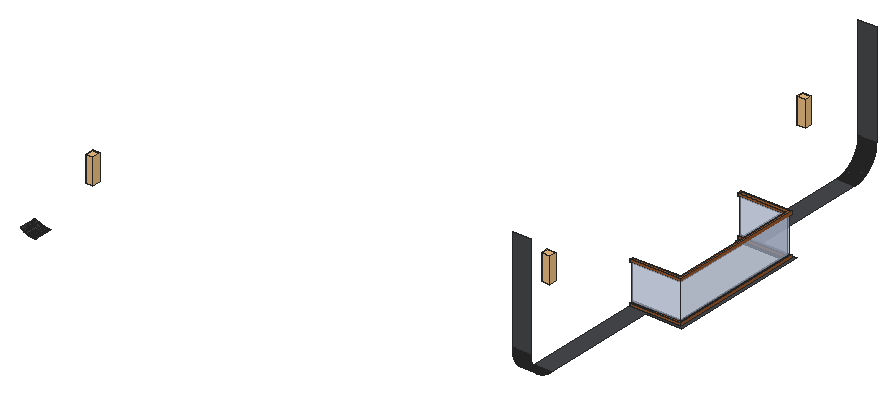
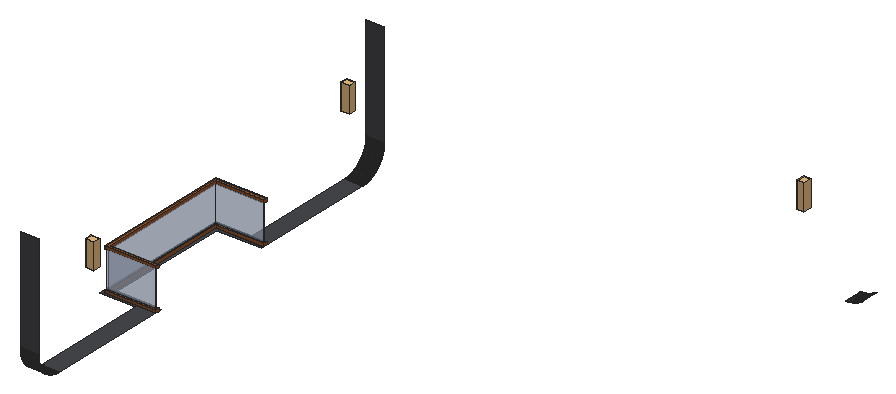
# SketchUp Ruby script. Lengths in inches.
U = 1.inch
M = Sketchup.active_model
def pt(a) = Geom::Point3d.new(a.map { |v| v * U })
def face(e, loops, mat)
  f = e.add_face(loops[0].map { |a| pt(a) })
  loops[1..].each { |l| e.add_face(l.map { |a| pt(a) }).erase! }
  f.material = f.back_material = mat if mat
  f
end
# faces: each face lists its corners as indices into pts; further lists are holes
def faces(e, pts, list, mat = nil) = list.each { |f| face(e, (f[0].is_a?(Array) ? f : [f]).map { |l| l.map { |i| pts[i] } }, mat) }
# xy, xz, yz: faces in a plane at the given z, y or x. An outline is a flat list of corners, or four numbers for a rectangle; further outlines are holes
def ring(l) = l.size == 4 ? [[l[0], l[1]], [l[2], l[1]], [l[2], l[3]], [l[0], l[3]]] : l.each_slice(2).to_a
def flat(e, list, mat, &to3) = list.each { |f| face(e, (f[0].is_a?(Array) ? f : [f]).map { |l| ring(l).map { |u, v| to3.(u, v) } }, mat) }
def xy(e, z, list, mat = nil) = flat(e, list, mat) { |x, y| [x, y, z] }
def xz(e, y, list, mat = nil) = flat(e, list, mat) { |x, z| [x, y, z] }
def yz(e, x, list, mat = nil) = flat(e, list, mat) { |y, z| [x, y, z] }
def lines(e, pts, list) = list.each { |a, b| e.add_line(pt(pts[a]), pt(pts[b])) }
# prism: a flat outline (further loops are holes) pulled along v
def prism(e, loops, v, mat = nil)
  f = face(e, loops, mat); d = Geom::Vector3d.new(v.map { |x| x * U })
  f.pushpull(f.normal.samedirection?(d) ? d.length : -d.length)
end
def box(e, o, s, mat = nil) = prism(e, [[o, [o[0] + s[0], o[1], o[2]], [o[0] + s[0], o[1] + s[1], o[2]], [o[0], o[1] + s[1], o[2]]]], [0, 0, s[2]], mat)
def at(x, y, z, deg = 0) = Geom::Transformation.translation(pt([x, y, z])) * Geom::Transformation.rotation(ORIGIN, Z_AXIS, deg.degrees)
def axes(o, x, y, z) = Geom::Transformation.new([*x, 0, *y, 0, *z, 0, *pt(o).to_a, 1])
def part(name) = M.definitions.add(name)
# library, detail: a bought-in or finely detailed component or shape, given as its bounding box
def library(name, o, s) = part(name).tap { |d| box(d.entities, o, s) }
def detail(e, o, s) = box(e.add_group.entities, o, s)
def put(e, d, t, mat = nil) = e.add_instance(d, t).tap { |i| i.material = mat if mat }
def group(e, t, mat = nil) = e.add_group.tap { |g| g.transformation = t; g.material = mat if mat }.entities
root = M.entities
M.materials.add("1432 AP 8245 TAR ROAD").color = [71, 72, 75]
M.materials.add("[Translucent Glass Blue]").color = [195, 208, 233]
M.materials["[Translucent Glass Blue]"].alpha = 0.5
M.materials.add("[Wood Cherry Original]").color = [152, 86, 42]
c1 = library("WALL LIGHT 69",[4.19,4.05,-8.78],[4.61,5.7,17.13])
c2 = part("Group\#47")
xy(c2.entities,0,[[0,0,0,2,32,2,32,90,0,90,0,92,34,92,34,0]])
xy(c2.entities,1.75,[[0.75,0.75,33.25,0.75,33.25,91.25,0.75,91.25,0.75,90.75,32.75,90.75,32.75,1.25,0.75,1.25]])
xy(c2.entities,2,[[[0,0,34,0,34,92,0,92,0,90,32,90,32,2,0,2],[0.75,0.75,0.75,1.25,32.75,1.25,32.75,90.75,0.75,90.75,0.75,91.25,33.25,91.25,33.25,0.75]]])
xy(c2.entities,26,[[[0,0,0,2,32,2,32,90,0,90,0,92,34,92,34,0],[0.75,0.75,33.25,0.75,33.25,91.25,0.75,91.25,0.75,90.75,32.75,90.75,32.75,1.25,0.75,1.25]]])
xy(c2.entities,26.25,[[0.75,0.75,0.75,1.25,32.75,1.25,32.75,90.75,0.75,90.75,0.75,91.25,33.25,91.25,33.25,0.75]])
xy(c2.entities,28,[[0,0,34,0,34,92,0,92,0,90,32,90,32,2,0,2]])
xz(c2.entities,0,[[0,0,34,2],[0,26,34,28]])
xz(c2.entities,0.75,[[0.75,1.75,33.25,2],[0.75,26,33.25,26.25]])
xz(c2.entities,1.25,[[0.75,1.75,32.75,2],[0.75,26,32.75,26.25]])
xz(c2.entities,2,[[0,0,32,2],[0,26,32,28]])
xz(c2.entities,90,[[0,0,32,2],[0,26,32,28]])
xz(c2.entities,90.75,[[0.75,1.75,32.75,2],[0.75,26,32.75,26.25]])
xz(c2.entities,91.25,[[0.75,1.75,33.25,2],[0.75,26,33.25,26.25]])
xz(c2.entities,92,[[0,0,34,2],[0,26,34,28]])
yz(c2.entities,0,[[0,0,2,2],[90,0,92,2],[0,26,2,28],[90,26,92,28]])
yz(c2.entities,0.75,[[0.75,1.75,1.25,2],[90.75,1.75,91.25,2],[0.75,26,1.25,26.25],[90.75,26,91.25,26.25]])
yz(c2.entities,32,[[2,0,90,2],[2,26,90,28]])
yz(c2.entities,32.75,[[1.25,1.75,90.75,2],[1.25,26,90.75,26.25]])
yz(c2.entities,33.25,[[0.75,1.75,91.25,2],[0.75,26,91.25,26.25]])
yz(c2.entities,34,[[0,0,92,2],[0,26,92,28]])
g1 = group(c2.entities,at(0.75,0.75,1.75),"[Translucent Glass Blue]")
prism(g1,[[[32,90,0],[0,90,0],[0,90.5,0],[32.5,90.5,0],[32.5,0,0],[0,0,0],[0,0.5,0],[32,0.5,0]]],[0,0,24.5])
xy(root,455.79,[[573,161.13,585,161.37],[573,161.37,585,161.37,585,239.37,609,239.37,609,335.37,585,335.37,585,413.37,573,413.37,573,329.37,603,329.37,603,245.37,573,245.37],[573,413.37,585,413.61]],"1432 AP 8245 TAR ROAD")
xy(root,461.79,[[293.76,95.37,294,107.37]],"1432 AP 8245 TAR ROAD")
xz(root,143.37,[[573,473.56,585,473.79],[573,473.79,585,542.79]],"1432 AP 8245 TAR ROAD")
xz(root,431.36,[[573,473.09,585,473.32]],"1432 AP 8245 TAR ROAD")
xz(root,431.37,[[573,473.56,585,473.79],[573,473.79,585,542.79]],"1432 AP 8245 TAR ROAD")
p = [[573,159.96,455.85],[573,159.72,455.87],[585,159.72,455.87],[585,159.96,455.85],[573,160.19,455.83],[585,160.19,455.83],
  [573,160.43,455.82],[585,160.43,455.82],[573,160.66,455.81],[585,160.66,455.81],[573,160.9,455.8],[585,160.9,455.8],
  [573,161.13,455.79],[585,161.13,455.79],[573,413.84,455.8],[573,413.61,455.79],[585,413.61,455.79],[585,413.84,455.8],
  [573,414.08,455.81],[585,414.08,455.81],[573,414.3125,455.82],[585,414.3125,455.82],[573,414.55,455.83],[585,414.55,455.83],
  [573,414.78,455.85],[585,414.78,455.85],[573,415.02,455.87],[585,415.02,455.87],[573,159.02,455.95],[573,158.79,455.98],
  [585,158.79,455.98],[585,159.02,455.95],[573,159.25,455.92],[585,159.25,455.92],[573,159.49,455.89],[585,159.49,455.89],
  [573,415.25,455.89],[585,415.25,455.89],[573,415.49,455.92],[585,415.49,455.92],[573,415.72,455.95],[585,415.72,455.95],
  [573,415.95,455.98],[585,415.95,455.98],[573,158.55,456.01],[573,158.32,456.05],[585,158.32,456.05],[585,158.55,456.01],
  [573,416.1875,456.01],[585,416.1875,456.01],[573,416.42,456.05],[585,416.42,456.05],[573,157.86,456.14],[573,157.63,456.19],
  [585,157.63,456.19],[585,157.86,456.14],[573,158.09,456.09],[585,158.09,456.09],[573,416.65,456.09],[585,416.65,456.09],
  [573,416.88,456.14],[585,416.88,456.14],[573,417.11,456.19],[585,417.11,456.19],[573,157.4,456.24],[573,157.17,456.29],
  [585,157.17,456.29],[585,157.4,456.24],[573,417.34,456.24],[585,417.34,456.24],[573,417.57,456.29],[585,417.57,456.29],
  [573,156.9375,456.35],[573,156.71,456.41],[585,156.71,456.41],[585,156.9375,456.35],[573,417.8,456.35],[585,417.8,456.35],
  [573,418.03,456.41],[585,418.03,456.41],[573,156.48,456.47],[585,156.48,456.47],[573,418.26,456.47],[585,418.26,456.47],
  [573,156.26,456.53],[573,156.03,456.6],[585,156.03,456.6],[585,156.26,456.53],[573,418.48,456.53],[585,418.48,456.53],
  [573,418.71,456.6],[585,418.71,456.6],[573,155.81,456.67],[585,155.81,456.67],[573,418.93,456.67],[585,418.93,456.67],
  [573,155.58,456.75],[573,155.36,456.82],[585,155.36,456.82],[585,155.58,456.75],[573,419.16,456.75],[585,419.16,456.75],
  [573,419.38,456.82],[585,419.38,456.82],[573,155.14,456.9],[585,155.14,456.9],[573,419.6,456.9],[585,419.6,456.9],
  [573,154.92,456.99],[585,154.92,456.99],[573,419.82,456.99],[585,419.82,456.99],[573,154.7,457.07],[585,154.7,457.07],
  [573,420.04,457.07],[585,420.04,457.07],[573,154.48,457.16],[585,154.48,457.16],[573,420.26,457.16],[585,420.26,457.16],
  [573,154.26,457.25],[585,154.26,457.25],[573,420.48,457.25],[585,420.48,457.25],[573,154.05,457.35],[573,153.83,457.45],
  [585,153.83,457.45],[585,154.05,457.35],[573,420.69,457.35],[585,420.69,457.35],[573,420.91,457.45],[585,420.91,457.45],
  [573,153.62,457.55],[585,153.62,457.55],[573,421.12,457.55],[585,421.12,457.55],[573,153.41,457.65],[585,153.41,457.65],
  [573,421.33,457.65],[585,421.33,457.65],[573,153.2,457.75],[585,153.2,457.75],[573,421.54,457.75],[585,421.54,457.75],
  [573,152.99,457.86],[585,152.99,457.86],[573,421.75,457.86],[585,421.75,457.86],[573,152.78,457.97],[585,152.78,457.97],
  [573,421.96,457.97],[585,421.96,457.97],[573,152.57,458.09],[585,152.57,458.09],[573,422.17,458.09],[585,422.17,458.09],
  [573,152.37,458.2],[585,152.37,458.2],[573,422.37,458.2],[585,422.37,458.2],[573,152.17,458.32],[585,152.17,458.32],
  [573,422.57,458.32],[585,422.57,458.32],[573,151.96,458.44],[585,151.96,458.44],[573,422.77,458.44],[585,422.77,458.44],
  [573,151.76,458.57],[585,151.76,458.57],[573,422.97,458.57],[585,422.97,458.57],[573,151.57,458.7],[585,151.57,458.7],
  [573,423.17,458.7],[585,423.17,458.7],[573,151.37,458.83],[585,151.37,458.83],[573,423.37,458.83],[585,423.37,458.83],
  [573,151.17,458.96],[585,151.17,458.96],[573,423.57,458.96],[585,423.57,458.96],[573,150.98,459.09],[585,150.98,459.09],
  [573,423.76,459.09],[585,423.76,459.09],[573,150.79,459.23],[585,150.79,459.23],[573,423.95,459.23],[585,423.95,459.23],
  [573,150.6,459.37],[585,150.6,459.37],[573,424.14,459.37],[585,424.14,459.37],[573,150.41,459.51],[585,150.41,459.51],
  [573,424.33,459.51],[585,424.33,459.51],[573,150.23,459.66],[585,150.23,459.66],[573,424.51,459.66],[585,424.51,459.66],
  [573,150.04,459.8],[585,150.04,459.8],[573,424.7,459.8],[585,424.7,459.8],[573,149.86,459.95],[585,149.86,459.95],
  [573,424.88,459.95],[585,424.88,459.95],[573,149.68,460.1],[585,149.68,460.1],[573,425.06,460.1],[585,425.06,460.1],
  [573,149.5,460.26],[585,149.5,460.26],[573,425.24,460.26],[585,425.24,460.26],[573,149.33,460.42],[585,149.33,460.42],
  [573,425.41,460.42],[585,425.41,460.42],[573,149.15,460.57],[585,149.15,460.57],[573,425.59,460.57],[585,425.59,460.57],
  [573,148.98,460.74],[585,148.98,460.74],[573,425.76,460.74],[585,425.76,460.74],[573,148.81,460.9],[585,148.81,460.9],
  [573,425.93,460.9],[585,425.93,460.9],[573,148.64,461.0625],[585,148.64,461.0625],[573,426.1,461.0625],[585,426.1,461.0625],
  [573,148.48,461.23],[585,148.48,461.23],[573,426.26,461.23],[585,426.26,461.23],[573,148.3125,461.4],[585,148.3125,461.4],
  [573,426.43,461.4],[585,426.43,461.4],[573,148.15,461.57],[585,148.15,461.57],[573,426.59,461.57],[585,426.59,461.57],
  [573,147.99,461.75],[585,147.99,461.75],[573,426.75,461.75],[585,426.75,461.75],[573,147.84,461.92],[585,147.84,461.92],
  [573,426.9,461.92],[585,426.9,461.92],[292.59,107.37,461.85],[292.35,107.37,461.87],[292.35,95.37,461.87],[292.59,95.37,461.85],
  [292.82,107.37,461.83],[292.82,95.37,461.83],[293.06,107.37,461.82],[293.06,95.37,461.82],[293.29,107.37,461.81],[293.29,95.37,461.81],
  [293.53,107.37,461.8],[293.53,95.37,461.8],[293.76,107.37,461.79],[293.76,95.37,461.79],[291.65,107.37,461.95],[291.42,107.37,461.98],
  [291.42,95.37,461.98],[291.65,95.37,461.95],[291.88,107.37,461.92],[291.88,95.37,461.92],[292.12,107.37,461.89],[292.12,95.37,461.89],
  [573,147.68,462.1],[585,147.68,462.1],[573,427.06,462.1],[585,427.06,462.1],[291.18,107.37,462.01],[290.95,107.37,462.05],
  [290.95,95.37,462.05],[291.18,95.37,462.01],[290.49,107.37,462.14],[290.26,107.37,462.19],[290.26,95.37,462.19],[290.49,95.37,462.14],
  [290.72,107.37,462.09],[290.72,95.37,462.09],[573,147.53,462.28],[585,147.53,462.28],[573,427.21,462.28],[585,427.21,462.28],
  [290.03,107.37,462.24],[289.8,107.37,462.29],[289.8,95.37,462.29],[290.03,95.37,462.24],[289.57,107.37,462.35],[289.34,107.37,462.41],
  [289.34,95.37,462.41],[289.57,95.37,462.35],[573,147.38,462.46],[585,147.38,462.46],[573,427.36,462.46],[585,427.36,462.46],
  [289.11,107.37,462.47],[289.11,95.37,462.47],[288.89,107.37,462.53],[288.66,107.37,462.6],[288.66,95.37,462.6],[288.89,95.37,462.53],
  [573,147.23,462.65],[585,147.23,462.65],[573,427.51,462.65],[585,427.51,462.65],[288.4375,107.37,462.67],[288.4375,95.37,462.67],
  [573,147.09,462.83],[585,147.09,462.83],[573,427.65,462.83],[585,427.65,462.83],[288.21,107.37,462.75],[287.99,107.37,462.82],
  [287.99,95.37,462.82],[288.21,95.37,462.75],[287.77,107.37,462.9],[287.77,95.37,462.9],[573,146.95,463.02],[585,146.95,463.02],
  [573,427.79,463.02],[585,427.79,463.02],[287.55,107.37,462.99],[287.55,95.37,462.99],[287.33,107.37,463.07],[287.33,95.37,463.07],
  [573,146.81,463.21],[585,146.81,463.21],[573,427.93,463.21],[585,427.93,463.21],[287.11,107.37,463.16],[287.11,95.37,463.16],
  [286.89,107.37,463.25],[286.89,95.37,463.25],[573,146.67,463.4],[585,146.67,463.4],[573,428.07,463.4],[585,428.07,463.4],
  [286.68,107.37,463.35],[286.46,107.37,463.45],[286.46,95.37,463.45],[286.68,95.37,463.35],[286.25,107.37,463.55],[286.25,95.37,463.55],
  [573,146.54,463.6],[585,146.54,463.6],[573,428.2,463.6],[585,428.2,463.6],[286.04,107.37,463.65],[286.04,95.37,463.65],
  [285.83,107.37,463.75],[285.83,95.37,463.75],[573,146.4,463.79],[585,146.4,463.79],[573,428.34,463.79],[585,428.34,463.79],
  [285.62,107.37,463.86],[285.62,95.37,463.86],[573,146.27,463.99],[585,146.27,463.99],[573,428.47,463.99],[585,428.47,463.99],
  [285.41,107.37,463.97],[285.41,95.37,463.97],[285.2,107.37,464.09],[285.2,95.37,464.09],[573,146.15,464.1875],[585,146.15,464.1875],
  [573,428.59,464.1875],[585,428.59,464.1875],[285,107.37,464.2],[285,95.37,464.2],[284.8,107.37,464.32],[284.8,95.37,464.32],
  [573,146.02,464.39],[585,146.02,464.39],[573,428.72,464.39],[585,428.72,464.39],[284.6,107.37,464.44],[284.6,95.37,464.44],
  [284.39,107.37,464.57],[284.39,95.37,464.57],[573,145.9,464.59],[585,145.9,464.59],[573,428.84,464.59],[585,428.84,464.59],
  [284.2,107.37,464.7],[284.2,95.37,464.7],[573,145.78,464.79],[585,145.78,464.79],[573,428.96,464.79],[585,428.96,464.79],
  [284,107.37,464.83],[284,95.37,464.83],[283.8,107.37,464.96],[283.8,95.37,464.96],[573,145.67,465],[585,145.67,465],
  [573,429.07,465],[585,429.07,465],[283.61,107.37,465.09],[283.61,95.37,465.09],[573,145.55,465.2],[585,145.55,465.2],
  [573,429.1875,465.2],[585,429.1875,465.2],[573,145.44,465.41],[585,145.44,465.41],[573,429.3,465.41],[585,429.3,465.41],
  [573,145.33,465.62],[585,145.33,465.62],[573,429.41,465.62],[585,429.41,465.62],[573,145.23,465.83],[585,145.23,465.83],
  [573,429.51,465.83],[585,429.51,465.83],[573,145.125,466.04],[585,145.125,466.04],[573,429.62,466.04],[585,429.62,466.04],
  [573,145.02,466.26],[585,145.02,466.26],[573,429.72,466.26],[585,429.72,466.26],[573,144.93,466.47],[585,144.93,466.47],
  [573,429.8125,466.47],[585,429.8125,466.47],[573,144.83,466.6875],[585,144.83,466.6875],[573,429.91,466.6875],[585,429.91,466.6875],
  [573,144.74,466.9],[585,144.74,466.9],[573,430,466.9],[585,430,466.9],[573,144.65,467.12],[585,144.65,467.12],
  [573,430.09,467.12],[585,430.09,467.12],[573,144.57,467.34],[585,144.57,467.34],[573,430.17,467.34],[585,430.17,467.34],
  [573,144.48,467.5625],[585,144.48,467.5625],[573,430.26,467.5625],[585,430.26,467.5625],[573,144.4,467.78],[585,144.4,467.78],
  [573,430.34,467.78],[585,430.34,467.78],[573,144.33,468.01],[585,144.33,468.01],[573,430.41,468.01],[585,430.41,468.01],
  [573,144.25,468.23],[585,144.25,468.23],[573,430.49,468.23],[585,430.49,468.23],[573,144.18,468.45],[585,144.18,468.45],
  [573,430.56,468.45],[585,430.56,468.45],[573,144.11,468.68],[585,144.11,468.68],[573,430.63,468.68],[585,430.63,468.68],
  [573,144.05,468.91],[585,144.05,468.91],[573,430.69,468.91],[585,430.69,468.91],[573,143.98,469.13],[585,143.98,469.13],
  [573,430.76,469.13],[585,430.76,469.13],[573,143.92,469.36],[585,143.92,469.36],[573,430.82,469.36],[585,430.82,469.36],
  [573,143.87,469.59],[585,143.87,469.59],[573,430.87,469.59],[585,430.87,469.59],[573,143.8125,469.82],[585,143.8125,469.82],
  [573,430.93,469.82],[585,430.93,469.82],[573,143.76,470.05],[585,143.76,470.05],[573,430.98,470.05],[585,430.98,470.05],
  [573,143.72,470.28],[585,143.72,470.28],[573,431.02,470.28],[585,431.02,470.28],[573,143.67,470.51],[585,143.67,470.51],
  [573,431.07,470.51],[585,431.07,470.51],[573,143.63,470.74],[585,143.63,470.74],[573,431.11,470.74],[585,431.11,470.74],
  [573,143.59,470.98],[585,143.59,470.98],[573,431.15,470.98],[585,431.15,470.98],[573,143.56,471.21],[585,143.56,471.21],
  [573,431.18,471.21],[585,431.18,471.21],[573,143.52,471.44],[585,143.52,471.44],[573,431.22,471.44],[585,431.22,471.44],
  [573,143.49,471.68],[585,143.49,471.68],[573,431.25,471.68],[585,431.25,471.68],[573,143.47,471.91],[585,143.47,471.91],
  [573,431.27,471.91],[585,431.27,471.91],[573,143.45,472.15],[585,143.45,472.15],[573,431.29,472.15],[585,431.29,472.15],
  [573,143.43,472.38],[585,143.43,472.38],[573,431.3125,472.38],[585,431.3125,472.38],[573,143.41,472.61],[585,143.41,472.61],
  [573,431.33,472.61],[585,431.33,472.61],[573,143.39,472.85],[585,143.39,472.85],[573,431.35,472.85],[585,431.35,472.85],
  [573,143.38,473.09],[585,143.38,473.09],[573,431.36,473.09],[585,431.36,473.09],[573,143.375,473.32],[585,143.375,473.32],
  [573,143.37,473.56],[585,143.37,473.56],[573,431.37,473.56],[573,431.36,473.32],[585,431.36,473.32],[585,431.37,473.56]]
faces(root,p,[[0,1,2,3],[4,0,3,5],[6,4,5,7],[8,6,7,9],[10,8,9,11],[12,10,11,13],[14,15,16,17],[18,14,17,19],
  [20,18,19,21],[22,20,21,23],[24,22,23,25],[26,24,25,27],[28,29,30,31],[32,28,31,33],[34,32,33,35],[1,34,35,2],
  [36,26,27,37],[38,36,37,39],[40,38,39,41],[42,40,41,43],[44,45,46,47],[29,44,47,30],[48,42,43,49],[50,48,49,51],
  [52,53,54,55],[56,52,55,57],[45,56,57,46],[58,50,51,59],[60,58,59,61],[62,60,61,63],[64,65,66,67],[53,64,67,54],
  [68,62,63,69],[70,68,69,71],[72,73,74,75],[65,72,75,66],[76,70,71,77],[78,76,77,79],[73,80,81,74],[82,78,79,83],
  [84,85,86,87],[80,84,87,81],[88,82,83,89],[90,88,89,91],[85,92,93,86],[94,90,91,95],[96,97,98,99],[92,96,99,93],
  [100,94,95,101],[102,100,101,103],[97,104,105,98],[106,102,103,107],[104,108,109,105],[110,106,107,111],[108,112,113,109],[114,110,111,115],
  [112,116,117,113],[118,114,115,119],[116,120,121,117],[122,118,119,123],[124,125,126,127],[120,124,127,121],[128,122,123,129],[130,128,129,131],
  [125,132,133,126],[134,130,131,135],[132,136,137,133],[138,134,135,139],[136,140,141,137],[142,138,139,143],[140,144,145,141],[146,142,143,147],
  [144,148,149,145],[150,146,147,151],[148,152,153,149],[154,150,151,155],[152,156,157,153],[158,154,155,159],[156,160,161,157],[162,158,159,163],
  [160,164,165,161],[166,162,163,167],[164,168,169,165],[170,166,167,171],[168,172,173,169],[174,170,171,175],[172,176,177,173],[178,174,175,179],
  [176,180,181,177],[182,178,179,183],[180,184,185,181],[186,182,183,187],[184,188,189,185],[190,186,187,191],[188,192,193,189],[194,190,191,195],
  [192,196,197,193],[198,194,195,199],[196,200,201,197],[202,198,199,203],[200,204,205,201],[206,202,203,207],[204,208,209,205],[210,206,207,211],
  [208,212,213,209],[214,210,211,215],[212,216,217,213],[218,214,215,219],[216,220,221,217],[222,218,219,223],[220,224,225,221],[226,222,223,227],
  [224,228,229,225],[230,226,227,231],[228,232,233,229],[234,230,231,235],[232,236,237,233],[238,234,235,239],[236,240,241,237],[242,238,239,243],
  [240,244,245,241],[246,242,243,247],[244,248,249,245],[250,246,247,251],[248,252,253,249],[254,250,251,255],[252,256,257,253],[258,254,255,259],
  [260,261,262,263],[264,260,263,265],[266,264,265,267],[268,266,267,269],[270,268,269,271],[272,270,271,273],[274,275,276,277],[278,274,277,279],
  [280,278,279,281],[261,280,281,262],[256,282,283,257],[284,258,259,285],[286,287,288,289],[275,286,289,276],[290,291,292,293],[294,290,293,295],
  [287,294,295,288],[282,296,297,283],[298,284,285,299],[300,301,302,303],[291,300,303,292],[304,305,306,307],[301,304,307,302],[296,308,309,297],
  [310,298,299,311],[305,312,313,306],[314,315,316,317],[312,314,317,313],[308,318,319,309],[320,310,311,321],[315,322,323,316],[318,324,325,319],
  [326,320,321,327],[328,329,330,331],[322,328,331,323],[329,332,333,330],[324,334,335,325],[336,326,327,337],[332,338,339,333],[338,340,341,339],
  [334,342,343,335],[344,336,337,345],[340,346,347,341],[346,348,349,347],[342,350,351,343],[352,344,345,353],[354,355,356,357],[348,354,357,349],
  [355,358,359,356],[350,360,361,351],[362,352,353,363],[358,364,365,359],[364,366,367,365],[360,368,369,361],[370,362,363,371],[366,372,373,367],
  [368,374,375,369],[376,370,371,377],[372,378,379,373],[378,380,381,379],[374,382,383,375],[384,376,377,385],[380,386,387,381],[386,388,389,387],
  [382,390,391,383],[392,384,385,393],[388,394,395,389],[394,396,397,395],[390,398,399,391],[400,392,393,401],[396,402,403,397],[398,404,405,399],
  [406,400,401,407],[402,408,409,403],[408,410,411,409],[404,412,413,405],[414,406,407,415],[410,416,417,411],[412,418,419,413],[420,414,415,421],
  [418,422,423,419],[424,420,421,425],[422,426,427,423],[428,424,425,429],[426,430,431,427],[432,428,429,433],[430,434,435,431],[436,432,433,437],
  [434,438,439,435],[440,436,437,441],[438,442,443,439],[444,440,441,445],[442,446,447,443],[448,444,445,449],[446,450,451,447],[452,448,449,453],
  [450,454,455,451],[456,452,453,457],[454,458,459,455],[460,456,457,461],[458,462,463,459],[464,460,461,465],[462,466,467,463],[468,464,465,469],
  [466,470,471,467],[472,468,469,473],[470,474,475,471],[476,472,473,477],[474,478,479,475],[480,476,477,481],[478,482,483,479],[484,480,481,485],
  [482,486,487,483],[488,484,485,489],[486,490,491,487],[492,488,489,493],[490,494,495,491],[496,492,493,497],[494,498,499,495],[500,496,497,501],
  [498,502,503,499],[504,500,501,505],[502,506,507,503],[508,504,505,509],[506,510,511,507],[512,508,509,513],[510,514,515,511],[516,512,513,517],
  [514,518,519,515],[520,516,517,521],[518,522,523,519],[524,520,521,525],[522,526,527,523],[528,524,525,529],[526,530,531,527],[532,528,529,533],
  [530,534,535,531],[536,532,533,537],[534,538,539,535],[540,536,537,541],[538,542,543,539],[544,540,541,545],[542,546,547,543],[548,544,545,549],
  [546,550,551,547],[552,548,549,553],[550,554,555,551],[556,552,553,557],[554,558,559,555],[560,556,557,561],[558,562,563,559],[562,564,565,563],
  [566,567,568,569]],"1432 AP 8245 TAR ROAD")
put(root,c1,at(319.46,95.62,512.4))
put(root,c1,at(583.25,162.99,511.97,90))
put(root,c2,at(573,241.37,455.79),"[Wood Cherry Original]")
put(root,c1,at(583.25,375.38,511.97,90))
